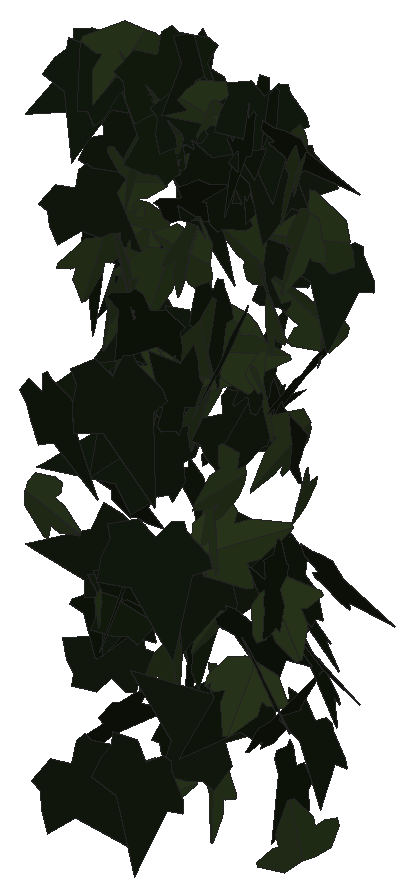
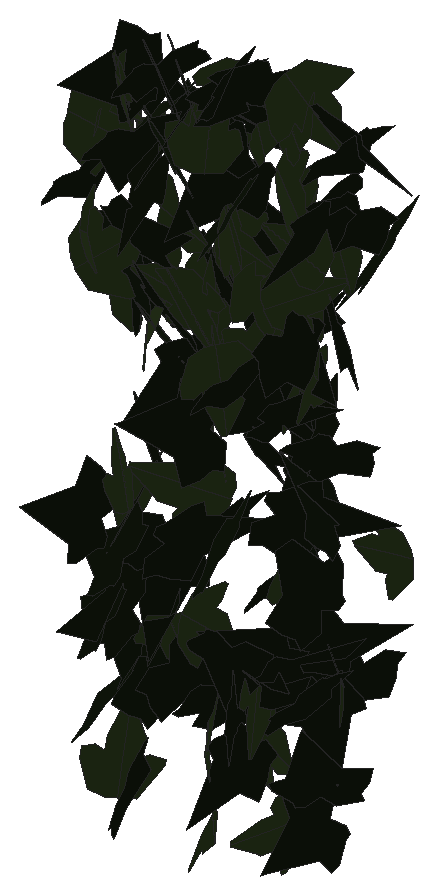
# SketchUp Ruby script. Lengths in inches.
U = 1.inch
M = Sketchup.active_model
def pt(a) = Geom::Point3d.new(a.map { |v| v * U })
def face(e, loops, mat)
  f = e.add_face(loops[0].map { |a| pt(a) })
  loops[1..].each { |l| e.add_face(l.map { |a| pt(a) }).erase! }
  f.material = f.back_material = mat if mat
  f
end
# faces: each face lists its corners as indices into pts; further lists are holes
def faces(e, pts, list, mat = nil) = list.each { |f| face(e, (f[0].is_a?(Array) ? f : [f]).map { |l| l.map { |i| pts[i] } }, mat) }
# xy, xz, yz: faces in a plane at the given z, y or x. An outline is a flat list of corners, or four numbers for a rectangle; further outlines are holes
def ring(l) = l.size == 4 ? [[l[0], l[1]], [l[2], l[1]], [l[2], l[3]], [l[0], l[3]]] : l.each_slice(2).to_a
def flat(e, list, mat, &to3) = list.each { |f| face(e, (f[0].is_a?(Array) ? f : [f]).map { |l| ring(l).map { |u, v| to3.(u, v) } }, mat) }
def xy(e, z, list, mat = nil) = flat(e, list, mat) { |x, y| [x, y, z] }
def xz(e, y, list, mat = nil) = flat(e, list, mat) { |x, z| [x, y, z] }
def yz(e, x, list, mat = nil) = flat(e, list, mat) { |y, z| [x, y, z] }
def lines(e, pts, list) = list.each { |a, b| e.add_line(pt(pts[a]), pt(pts[b])) }
# prism: a flat outline (further loops are holes) pulled along v
def prism(e, loops, v, mat = nil)
  f = face(e, loops, mat); d = Geom::Vector3d.new(v.map { |x| x * U })
  f.pushpull(f.normal.samedirection?(d) ? d.length : -d.length)
end
def box(e, o, s, mat = nil) = prism(e, [[o, [o[0] + s[0], o[1], o[2]], [o[0] + s[0], o[1] + s[1], o[2]], [o[0], o[1] + s[1], o[2]]]], [0, 0, s[2]], mat)
def at(x, y, z, deg = 0) = Geom::Transformation.translation(pt([x, y, z])) * Geom::Transformation.rotation(ORIGIN, Z_AXIS, deg.degrees)
def axes(o, x, y, z) = Geom::Transformation.new([*x, 0, *y, 0, *z, 0, *pt(o).to_a, 1])
def part(name) = M.definitions.add(name)
# library, detail: a bought-in or finely detailed component or shape, given as its bounding box
def library(name, o, s) = part(name).tap { |d| box(d.entities, o, s) }
def detail(e, o, s) = box(e.add_group.entities, o, s)
def put(e, d, t, mat = nil) = e.add_instance(d, t).tap { |i| i.material = mat if mat }
def group(e, t, mat = nil) = e.add_group.tap { |g| g.transformation = t; g.material = mat if mat }.entities
root = M.entities
M.materials.add("efeu1").color = [18, 25, 13]
M.materials.add("efeu2").color = [43, 57, 29]
c1 = part("ivyleaf_9")
p = [[1.54,2.16,1.25],[1.36,2.04,1.19],[-0.21,0.99,0.68],[-0.71,1.11,0.82],[-0.85,0.86,0.67],[-0.8,0.17,0.21],
  [-0.9,-0.01,0.1],[-0.67,-0.16,-0.02],[-0.08,-0.08,-0.05],[-0.03,-0.6,-0.4],[0.65,-0.88,-0.66],[0.83,-0.6,-0.49],
  [1.29,-0.42,-0.43],[1.8125,-0.07,-0.26],[1.21,0.44,0.15]]
faces(c1.entities,p,[[0,1,2,3,4,5,6,7,8,9,10,11,12,13,14]],"efeu1")
c2 = part("ivyleaf_10")
p = [[0,0.5,-0.03],[-0.0625,2.02,-0.43],[-0.19,2.01,-0.46],[-0.54,1.05,-0.29],[-0.52,0.625,-0.18],[-0.83,0.76,-0.28],
  [-1.16,0.64,-0.33],[-1.15,0.33,-0.24],[-0.77,-0.39,0.02],[-0.3,-0.51,0.16],[0.04,-0.48,0.23],[-0.02,2.01,-0.4375],
  [-0.06,2.01,-0.43],[0.04,-0.49,0.23],[0.67,-0.49,0.14],[1.38,0.36,-0.2],[1.375,0.51,-0.24],[0.81,0.65,-0.19],
  [0.62,0.59,-0.15],[0.6,1.09,-0.28],[0.5,1.23,-0.31]]
faces(c2.entities,p,[[0,1,2,3,4,5,6,7,8,9,10],[11,12,0,13,14,15,16,17,18,19,20]],"efeu2")
put(root,c1,axes([549.42,123.8,195.95],[-0.57718,-0.61121,-0.72388],[0.47764,0.5443,-0.84042],[0.81819,-0.74891,-0.02003]))
put(root,c1,axes([548.41,124.625,188.24],[-0.02119,-1.07026,0.20723],[-0.00657,-0.20714,-1.07047],[1.09012,-0.02205,-0.00242]))
put(root,c1,axes([545.25,124.21,198.84],[0.70279,-0.78365,-0.25205],[-0.16067,0.19446,-1.05258],[0.80736,0.72085,0.00994]))
put(root,c1,axes([547.02,125.02,199.58],[0.33502,-1.12764,-0.34099],[-0.05541,0.33903,-1.17561],[1.17676,0.337,0.04172]))
put(root,c1,axes([545.31,125.4,186.8125],[0.2181,-0.64574,-0.82159],[-0.13191,0.81557,-0.67602],[1.03662,0.23964,0.08683]))
put(root,c1,axes([550.37,126.05,201.71],[-0.61708,0.48349,-0.48625],[0.38738,-0.29397,-0.78391],[-0.56581,-0.72857,-0.00639]))
put(root,c1,axes([545.82,127.31,197.32],[-0.2236,-0.7327,0.45613],[-0.14148,-0.4337,-0.76602],[0.8514,-0.26449,-0.0075]))
put(root,c1,axes([548.18,126.54,198.61],[-0.24274,0.35449,0.80046],[-0.44067,0.66827,-0.42959],[-0.75645,-0.50306,-0.00661]))
put(root,c1,axes([546.37,127.35,200.48],[0.36131,0.27193,-0.7739],[-0.62588,-0.45523,-0.45216],[-0.53023,0.72266,0.00638]))
put(root,c2,axes([546.47,127.98,185.49],[0.3402,-0.69061,0.64263],[0.24333,-0.59578,-0.76908],[0.91143,0.41684,-0.03454]))
put(root,c2,axes([545.1,127.73,201.73],[-0.50619,0.63955,-0.34988],[0.20413,-0.28456,-0.81548],[-0.69983,-0.54559,0.0152]))
put(root,c2,axes([550.5,128.54,197.58],[0.10546,-0.42785,0.89084],[0.16836,-0.87502,-0.44019],[0.97381,0.19762,-0.02037]))
put(root,c2,axes([549.6,128.42,201.43],[-0.13056,-0.06951,1.03991],[0.93887,-0.46289,0.08693],[0.45252,0.94032,0.11967]))
put(root,c2,axes([543.94,128.16,201.28],[-0.2056,-0.84361,0.13688],[-0.0284,-0.13396,-0.8683],[0.85417,-0.20752,0.00408]))
put(root,c1,axes([545.15,128.37,192.2],[-0.60065,0.31014,-0.74291],[0.6392,-0.37977,-0.67534],[-0.48942,-0.87663,0.02973]))
put(root,c1,axes([550.5625,127.74,193.1875],[-0.26872,0.05826,-0.9062],[-0.90137,0.09747,0.27355],[0.1101,0.94016,0.0278]))
put(root,c2,axes([541.73,128.35,192.64],[-0.21275,0.09277,-0.83059],[0.76162,-0.33137,-0.2321],[-0.34411,-0.79078,-0.00018]))
put(root,c2,axes([548.03,128.88,195.17],[-0.02013,0.03747,0.8963],[0.24819,-0.8613,0.04159],[0.86207,0.24884,0.00896]))
put(root,c1,axes([549.93,128.68,197.26],[0.01773,-0.02831,0.98933],[0.41915,-0.89616,-0.03315],[0.89659,0.4195,-0.00406]))
put(root,c2,axes([547.42,128.7,194.13],[0.45083,-0.35978,0.67627],[0.60292,-0.31739,-0.57078],[0.47252,0.74824,0.08306]))
put(root,c1,axes([547.11,129,191.95],[-0.16652,-0.83164,0.26203],[-0.05383,-0.25646,-0.84814],[0.87028,-0.17498,-0.00232]))
put(root,c2,axes([549.85,128.52,192.17],[0.29451,0.80983,0.27461],[0.10574,0.25372,-0.86164],[-0.84856,0.31269,-0.01206]))
put(root,c1,axes([543.57,129.5,195.7],[0.16315,-0.48763,0.92572],[0.42472,-0.82538,-0.50963],[0.95622,0.4498,0.06841]))
put(root,c2,axes([550.24,129.34,203.55],[-0.00457,0.65938,-0.65939],[-0.07106,-0.65773,-0.65722],[-0.9298,0.04702,0.05347]))
put(root,c1,axes([547.26,129.32,186.6],[-0.47495,-0.94187,-0.19726],[-0.08698,-0.17706,1.05485],[-0.95837,0.48285,0.00202]))
put(root,c2,axes([547.02,128.72,199.57],[0.02035,-0.99592,-0.42809],[0.06292,0.42852,-0.99395],[1.0822,-0.00619,0.06584]))
put(root,c1,axes([550.5,128.76,199.34],[-0.35348,0.83089,-0.13837],[0.05656,-0.1263,-0.90296],[-0.84044,-0.35797,-0.00257]))
put(root,c1,axes([542.8125,128.6875,202.4375],[0.03003,-0.35847,-0.79405],[0.18655,0.77874,-0.3445],[0.85101,-0.15806,0.10354]))
put(root,c2,axes([545.77,129.14,197.55],[0.45462,0.63733,0.38042],[-0.22565,-0.30632,0.78284],[0.7071,-0.50751,0.00524]))
put(root,c1,axes([548.42,129.58,189.05],[0.64388,-0.25384,-0.75639],[0.73295,-0.19579,0.68964],[-0.31519,-0.97385,0.05851]))
put(root,c2,axes([546.75,129.28,197.23],[0.25038,-0.88746,0.00656],[0.00178,-0.00631,-0.9221],[0.88748,0.25039,0]))
put(root,c2,axes([548.63,129.84,197.34],[-0.27187,-0.16957,1.02457],[0.82041,-0.68442,0.10443],[0.63673,0.80946,0.30292]))
put(root,c1,axes([548.71,128.97,190.83],[0.8061,0.39429,-0.53653],[-0.49134,-0.21633,-0.89717],[-0.44936,0.94385,0.01851]))
put(root,c1,axes([546.1,129.05,195.01],[-0.58985,0.00585,-0.65301],[-0.65302,-0.01087,0.58976],[-0.00415,0.8799,0.01163]))
put(root,c1,axes([548.9,129.17,197.14],[-0.66653,0.56479,0.32275],[-0.25495,0.19832,-0.87354],[-0.59846,-0.71351,0.01268]))
put(root,c2,axes([549.8,129.71,183.92],[-0.4319,-0.82846,-0.30957],[-0.14869,-0.27159,0.93426],[-0.87182,0.45674,-0.00598]))
put(root,c1,axes([547.84,129.93,188],[-0.04498,0.08958,-0.88875],[0.09631,-0.88421,-0.094],[-0.88805,-0.10043,0.03482]))
put(root,c2,axes([548.1,129.5,188.84],[0.7964,0.3624,-0.22264],[-0.20307,-0.09129,-0.87498],[-0.37372,0.82188,0.00098]))
put(root,c1,axes([546.73,129.63,200.14],[-0.47231,-0.013,-0.75126],[0.74805,0.07519,-0.47159],[0.07056,-0.8842,-0.02906]))
put(root,c2,axes([547.35,129,192.78],[0.28135,0.15131,-1.02625],[0.95694,0.37262,0.31728],[0.40045,-0.99675,-0.03717]))
put(root,c2,axes([544.72,128.87,184],[0.00323,-0.05009,-0.94639],[0.46591,0.82421,-0.04203],[0.82528,-0.46512,0.02743]))
put(root,c2,axes([544.91,129.85,204.34],[-0.51817,0.08628,0.76506],[0.71505,-0.28793,0.51677],[0.28541,0.87802,0.09429]))
put(root,c1,axes([546.59,129.65,203.05],[-0.30607,0.12731,0.95543],[0.78657,-0.54641,0.32478],[0.55711,0.8414,0.06636]))
put(root,c1,axes([545.61,129.61,204.48],[-0.78533,-0.31379,-0.39363],[-0.36477,-0.14797,0.84569],[-0.34692,0.8659,0.00187]))
put(root,c2,axes([547.38,129.5,198.59],[-0.26753,-0.08974,0.92934],[0.86763,0.33321,0.28194],[-0.34489,0.90786,-0.01162]))
put(root,c2,axes([542.27,130.13,189.49],[-0.245,0.13324,-0.80396],[0.39356,-0.71577,-0.23856],[-0.71359,-0.4405,0.14446]))
put(root,c1,axes([547.65,129.96,205.66],[-0.59116,0.16505,-0.63443],[0.619,-0.14072,-0.61339],[-0.21583,-0.85567,-0.0215]))
put(root,c1,axes([544.43,129.66,197.05],[-0.16886,-0.28061,-0.80655],[0.57072,0.5745,-0.31936],[0.63524,-0.59074,0.07253]))
put(root,c1,axes([544.26,129.96,197.67],[-0.51379,-0.11989,-0.67977],[0.66915,0.12147,-0.52719],[0.16942,-0.8434,0.0207]))
put(root,c2,axes([547.67,129.81,199.09],[0.94163,-0.26869,-0.48567],[-0.46848,0.12818,-0.97921],[0.29766,1.05172,-0.00474]))
put(root,c1,axes([542.83,129.93,205.63],[-0.94114,0.20242,0.21658],[-0.21279,0.04066,-0.96265],[-0.20641,-0.96488,0.00487]))
put(root,c2,axes([544.38,129.56,191.35],[-0.69811,0.47864,0.18463],[-0.15641,0.09836,-0.84641],[-0.48859,-0.71539,0.00716]))
put(root,c1,axes([547.46,130.5625,191.95],[-0.0877,-0.5801,-0.82183],[-0.00619,-0.82462,0.58273],[-1.00592,0.05565,0.06806]))
put(root,c1,axes([547.48,129.26,196.82],[0.11196,-0.12772,-0.87621],[-0.07688,0.87845,-0.13787],[0.88213,0.09277,0.09919]))
put(root,c1,axes([542.09,130.4,205.17],[-0.2167,-0.89598,0.17583],[-0.01535,-0.17711,-0.92144],[0.91294,-0.21565,0.02625]))
put(root,c1,axes([542.69,129.75,196.0625],[-0.00809,-0.61205,-0.66691],[0.29456,0.62885,-0.5807],[0.85592,-0.22221,0.19354]))
put(root,c2,axes([544.8,130.01,200.37],[-0.4589,-0.85692,0.21949],[-0.08982,-0.20085,-0.97194],[0.88001,-0.46736,0.01525]))
put(root,c2,axes([543.53,130.24,197.78],[-0.09499,0.57564,-0.62708],[-0.04518,-0.6335,-0.57469],[-0.85003,-0.03066,0.10062]))
put(root,c1,axes([548.11,129.52,197.67],[-0.59829,0.58624,0.31908],[0.23823,-0.21271,0.83752],[0.62348,0.64383,-0.01383]))
put(root,c1,axes([543.85,130.52,194.02],[-0.1656,-0.43447,-0.95328],[-0.33333,-0.8931,0.46495],[-0.99317,0.37219,0.0029]))
put(root,c1,axes([542.93,130.32,190.31],[-0.28822,-0.10694,0.83485],[-0.79409,-0.25797,-0.30719],[0.279,-0.84469,-0.01188]))
put(root,c1,axes([546.05,129.29,203.0625],[0.76235,0.56155,0.23401],[0.17765,0.15332,-0.94668],[-0.58184,0.78258,0.01756]))
put(root,c2,axes([543.46,130.34,206.51],[-0.44485,-0.74037,0.57588],[-0.13923,-0.57818,-0.85089],[0.92758,-0.44186,0.14846]))
put(root,c1,axes([549.03,130.68,191.78],[0.49226,-0.85042,-0.4558],[0.35873,-0.31371,0.97273],[-0.89571,-0.59301,0.13908]))
put(root,c2,axes([543.55,130.21,205.08],[-0.41986,0.00825,0.84409],[0.81471,-0.24275,0.40762],[0.22091,0.91096,0.10098]))
put(root,c2,axes([545.71,130.14,201.63],[0.23727,-1.0565,0.06794],[0.0206,-0.06501,-1.0828],[1.05848,0.23809,0.00584]))
put(root,c2,axes([550.59,130.125,203],[-0.15878,-0.08567,1.02244],[-0.95767,-0.35892,-0.17879],[0.36821,-0.97045,-0.02413]))
put(root,c2,axes([544,129.33,200.04],[-0.04446,-0.56041,-0.90692],[0.0773,0.90362,-0.56216],[1.06329,-0.08913,0.00295]))
put(root,c1,axes([548.54,129.73,186.98],[0.20233,0.86361,0.15474],[-0.04888,-0.14746,0.88689],[0.876,-0.20769,0.01375]))
put(root,c1,axes([548.1,130.62,204.05],[-0.09929,-0.82758,0.41164],[0.17669,-0.42337,-0.80854],[0.90726,-0.00812,0.20251]))
put(root,c2,axes([543.78,130.37,203.72],[0.41565,-0.86728,0.37533],[0.19241,-0.32378,-0.96123],[0.92522,0.45695,0.03128]))
put(root,c2,axes([546.12,129.89,200.98],[0.00617,0.03823,0.95902],[-0.95928,-0.03073,0.0074],[0.031,-0.95855,0.03801]))
put(root,c1,axes([542.13,130.33,200.14],[-0.47327,0.03178,-0.81915],[0.81586,-0.07392,-0.47424],[-0.07989,-0.94315,0.00957]))
put(root,c1,axes([542.78,129.79,193.85],[-0.05693,0.81888,0.22225],[0.01126,-0.222,0.82085],[0.84843,0.05789,0.00402]))
put(root,c2,axes([548.95,130.53,204.89],[0.42482,-0.62316,0.5523],[0.3382,-0.43745,-0.75371],[0.76091,0.54235,0.02665]))
put(root,c2,axes([545.02,129.87,188.55],[0.06508,-0.91263,-0.40148],[0.04217,0.4045,-0.91265],[0.99615,0.0425,0.06487]))
put(root,c1,axes([543.01,129.96,189],[0.43399,0.43734,-0.60466],[-0.43698,-0.41808,-0.61603],[-0.60492,0.61577,0.0112]))
put(root,c1,axes([549.1,130.47,190.93],[0.3952,-0.64198,0.51276],[0.35268,-0.38135,-0.74928],[0.74207,0.52314,0.08304]))
put(root,c1,axes([545.7,129.96,205.64],[0.01976,-0.57226,-0.67125],[0.07119,0.67026,-0.56932],[0.8792,-0.04142,0.06119]))
put(root,c2,axes([546.16,130.2,197.51],[-0.55472,-0.75141,0.09476],[-0.05042,-0.08056,-0.93396],[0.75568,-0.55696,0.00725]))
put(root,c2,axes([545.86,129.83,205.72],[-0.44045,-0.41984,-0.64128],[0.51491,0.3858,-0.60624],[0.56778,-0.67557,0.05233]))
put(root,c1,axes([543.79,130.43,189.19],[-0.53776,-0.71068,-0.22726],[-0.1356,-0.18238,0.8912],[-0.7337,0.55459,0.00186]))
put(root,c2,axes([546.43,130.8,190.15],[0.00449,-0.56231,0.70081],[0.08279,-0.69758,-0.56025],[0.89469,0.06737,0.04832]))
put(root,c2,axes([542.67,130.6,198.51],[-0.11448,0.62524,-0.58106],[0.03238,-0.58266,-0.63334],[-0.85293,-0.10603,0.05395]))
put(root,c1,axes([543.48,129.99,189.43],[0.32295,0.00178,0.93752],[0.9375,-0.00819,-0.32293],[0.00717,0.99155,-0.00435]))
put(root,c1,axes([550.13,130.84,202.08],[-0.1024,-0.94627,0.07143],[-0.00499,-0.0713,-0.95179],[0.94895,-0.10248,0.0027]))
put(root,c2,axes([549.87,130.89,200.38],[0.30956,-0.37685,0.75157],[0.48429,-0.57476,-0.48767],[0.68727,0.57475,0.00511]))
put(root,c1,axes([548.54,130.27,205.2],[0.73856,-0.2124,0.4587],[0.44318,-0.11856,-0.76846],[0.24314,0.86129,0.00734]))
put(root,c1,axes([549.33,130.86,189.15],[0.32622,-0.63434,0.56384],[0.23404,-0.5134,-0.713],[0.8158,0.40094,-0.02092]))
put(root,c1,axes([544.5,130.17,206.5],[0.176,-0.63563,-0.80748],[0.27388,0.81862,-0.5847],[0.99047,-0.11341,0.30516]))
put(root,c1,axes([545.13,130.87,188.39],[-0.16134,0.10146,-0.94552],[0.84452,-0.42558,-0.18977],[-0.43716,-0.85961,-0.01765]))
put(root,c1,axes([545.41,131.14,206.03],[-0.1732,-0.53915,0.67346],[-0.17981,-0.64925,-0.56602],[0.84374,-0.24904,0.01762]))
put(root,c2,axes([546.16,130.75,203.94],[-0.41404,-0.84784,-0.28024],[-0.11572,-0.25534,0.94351],[-0.88542,0.42984,0.00773]))
put(root,c2,axes([549.16,130.41,205.125],[0.53819,-0.65135,-0.26115],[-0.14536,0.21849,-0.84454],[0.68654,0.55688,0.0259]))
put(root,c1,axes([545.35,131.21,192.52],[0.16956,-0.75576,0.7426],[0.14151,-0.72916,-0.77439],[1.05005,0.22031,-0.01556]))
put(root,c1,axes([545.34,130.6875,202.41],[0.51174,-0.79217,0.0087],[0.00472,-0.0073,-0.94309],[0.79221,0.51176,0]))
put(root,c2,axes([545.91,130.82,184.5625],[-0.17782,0.74198,-0.6107],[0.16487,-0.58831,-0.76277],[-0.94674,-0.24181,-0.01812]))
put(root,c1,axes([547.61,130.79,205.98],[-0.08188,-0.91483,-0.23042],[0.02998,0.22865,-0.91844],[0.94293,-0.08671,0.00919]))
put(root,c2,axes([543.57,130.84,200.51],[-0.27583,-0.08442,-0.81615],[-0.75657,-0.30706,0.28746],[-0.31755,0.80492,0.02406]))
put(root,c2,axes([545.72,131.08,186.77],[0.01321,-0.14029,0.93823],[0.73933,-0.58644,-0.0981],[0.59444,0.73249,0.10115]))
put(root,c1,axes([549.08,131.16,186.97],[0.1768,-0.87178,0.44567],[0.14104,-0.42548,-0.88823],[0.96888,0.22102,0.04797]))
put(root,c1,axes([545.08,131.04,197.78],[-0.08584,-0.92638,0.02959],[0.0025,-0.02995,-0.93033],[0.92685,-0.08572,0.00525]))
put(root,c2,axes([547.67,130.375,201.38],[0.05628,-0.01039,0.99452],[-0.98641,0.12679,0.05715],[-0.12718,-0.98801,-0.00313]))
put(root,c2,axes([542.71,130.57,201.81],[-0.31066,-0.11348,0.79513],[0.77733,0.17213,0.32827],[-0.20219,0.83613,0.04034]))
put(root,c1,axes([547.61,130.91,205.98],[-0.63144,0.09243,-0.60215],[0.59252,-0.10835,-0.63798],[-0.14156,-0.86577,0.01556]))
put(root,c1,axes([549.65,130.75,192.03],[0.63427,-0.34664,0.57854],[0.5036,-0.28486,-0.72278],[0.44862,0.80985,-0.0066]))
put(root,c1,axes([545.31,130.07,186.46],[0.0063,-0.07492,-0.88045],[-0.33428,0.81483,-0.07173],[0.81796,0.33358,-0.02253]))
put(root,c1,axes([542.33,130.85,192.01],[0.84876,0.03663,-0.41211],[0.40624,0.10441,0.84596],[0.07838,-0.93773,0.07809]))
put(root,c2,axes([549.76,130.83,199.61],[-0.62465,0.0604,-0.75787],[-0.7601,-0.02901,0.62418],[0.01597,0.98168,0.06508]))
put(root,c1,axes([542.73,130.04,185.27],[0.35851,0.56861,0.52911],[0.26565,0.45785,-0.67202],[-0.72987,0.44594,0.01531]))
put(root,c1,axes([548.6,130.77,189.71],[0.76009,-0.39648,0.29598],[0.26234,-0.13706,-0.85728],[0.4195,0.80409,-0.00018]))
put(root,c1,axes([542.58,131.44,189.36],[-0.23174,-0.86592,0.27709],[-0.0448,-0.27473,-0.896],[0.90807,-0.23453,0.02651]))
put(root,c1,axes([543.5,131.45,197.31],[-0.44709,-0.43393,0.52991],[-0.31822,-0.42876,-0.61959],[0.60649,-0.54485,0.06554]))
put(root,c1,axes([547.08,131.52,203.85],[0.02053,-0.73537,0.56993],[-0.00933,-0.57021,-0.73539],[0.93033,0.01051,-0.01995]))
put(root,c1,axes([546.61,130.12,195.42],[-0.02115,0.76391,-0.54859],[-0.05132,0.54697,0.76363],[0.93908,0.04709,0.02938]))
put(root,c1,axes([548.55,130.7,200.68],[-0.13839,0.22561,0.8065],[-0.7033,0.41247,-0.23607],[-0.45465,-0.70673,0.11968]))
put(root,c1,axes([547.54,131.04,204.28],[-0.71777,0.27318,-0.35069],[0.33849,-0.09588,-0.76749],[-0.28816,-0.79309,-0.02801]))
put(root,c1,axes([544.94,131.1,189.95],[-0.62466,-0.44863,-0.62446],[0.50278,0.37041,-0.76905],[0.58175,-0.80184,-0.00587]))
put(root,c1,axes([548.07,131.54,185.01],[0.18204,-0.15233,-0.90399],[0.70863,-0.56132,0.23729],[-0.58159,-0.73162,0.00616]))
put(root,c1,axes([542.44,130.65,186.42],[-0.70717,-0.19351,0.53672],[0.5193,0.13572,0.73315],[-0.23631,0.87735,0.00496]))
put(root,c1,axes([548.09,131.16,204],[-0.13368,-0.94281,-0.35649],[0.09931,0.34554,-0.9511],[1.00305,-0.15987,0.04666]))
put(root,c1,axes([542.39,130.46,203.2],[0.26723,-0.26495,-0.76338],[-0.24083,0.74139,-0.34162],[0.77133,0.32328,0.15781]))
put(root,c2,axes([548.5,131.14,193.29],[0.2737,-0.76664,-0.23931],[0.08107,-0.22515,0.81403],[-0.79902,-0.28545,0.00062]))
put(root,c1,axes([547.8,130.71,203.04],[0.74675,-0.11122,-0.47303],[-0.46545,0.08547,-0.75487],[0.13961,0.87983,0.01353]))
put(root,c1,axes([543.11,131.27,199.77],[-0.18325,0.46361,-0.69577],[0.21835,-0.66103,-0.49797],[-0.80706,-0.28411,0.02325]))
